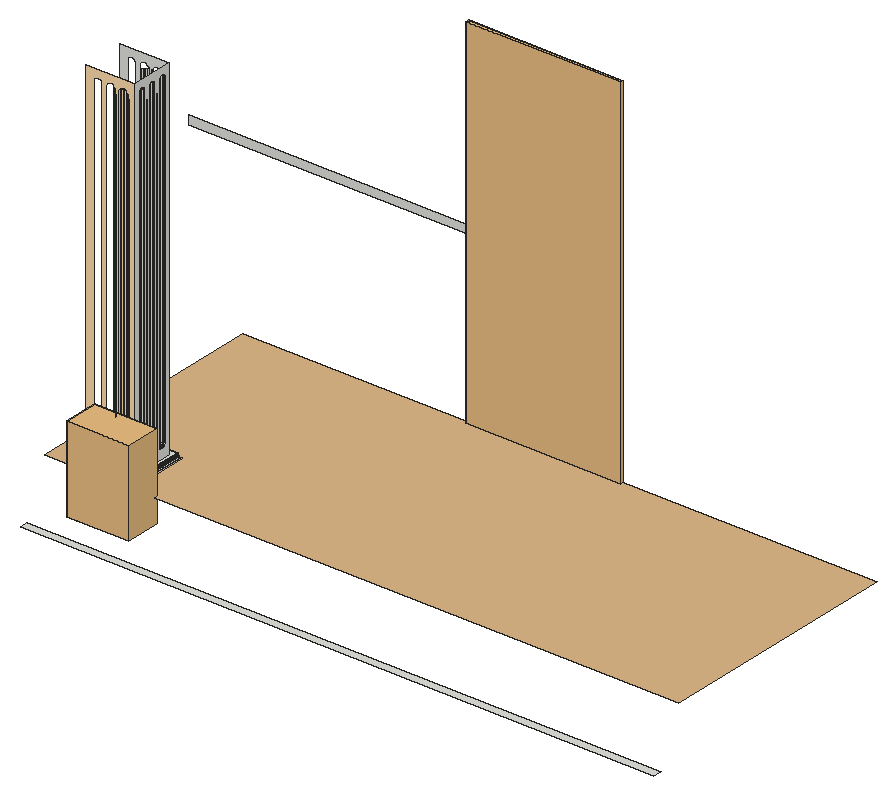
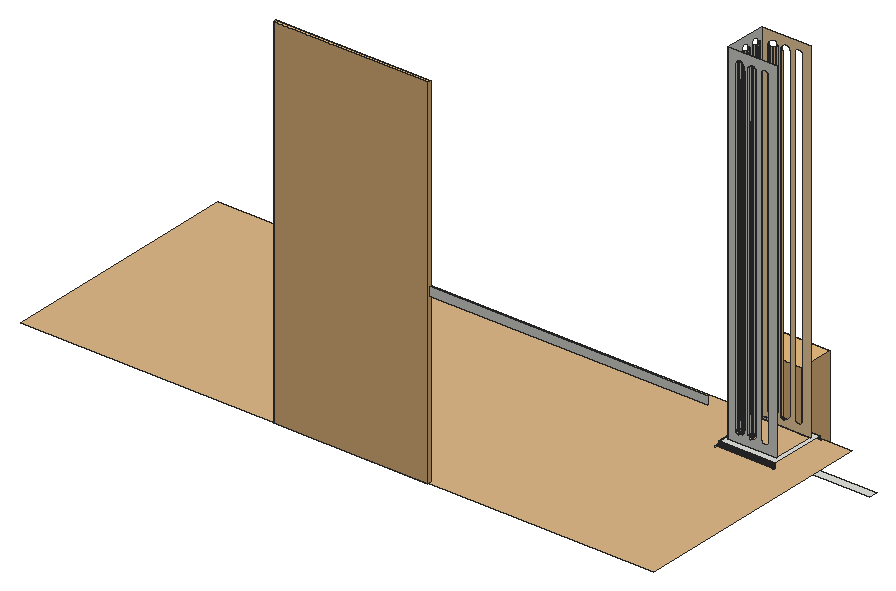
# SketchUp Ruby script. Lengths in inches.
U = 1.inch
M = Sketchup.active_model
def pt(a) = Geom::Point3d.new(a.map { |v| v * U })
def face(e, loops, mat)
  f = e.add_face(loops[0].map { |a| pt(a) })
  loops[1..].each { |l| e.add_face(l.map { |a| pt(a) }).erase! }
  f.material = f.back_material = mat if mat
  f
end
# faces: each face lists its corners as indices into pts; further lists are holes
def faces(e, pts, list, mat = nil) = list.each { |f| face(e, (f[0].is_a?(Array) ? f : [f]).map { |l| l.map { |i| pts[i] } }, mat) }
# xy, xz, yz: faces in a plane at the given z, y or x. An outline is a flat list of corners, or four numbers for a rectangle; further outlines are holes
def ring(l) = l.size == 4 ? [[l[0], l[1]], [l[2], l[1]], [l[2], l[3]], [l[0], l[3]]] : l.each_slice(2).to_a
def flat(e, list, mat, &to3) = list.each { |f| face(e, (f[0].is_a?(Array) ? f : [f]).map { |l| ring(l).map { |u, v| to3.(u, v) } }, mat) }
def xy(e, z, list, mat = nil) = flat(e, list, mat) { |x, y| [x, y, z] }
def xz(e, y, list, mat = nil) = flat(e, list, mat) { |x, z| [x, y, z] }
def yz(e, x, list, mat = nil) = flat(e, list, mat) { |y, z| [x, y, z] }
def lines(e, pts, list) = list.each { |a, b| e.add_line(pt(pts[a]), pt(pts[b])) }
# prism: a flat outline (further loops are holes) pulled along v
def prism(e, loops, v, mat = nil)
  f = face(e, loops, mat); d = Geom::Vector3d.new(v.map { |x| x * U })
  f.pushpull(f.normal.samedirection?(d) ? d.length : -d.length)
end
def box(e, o, s, mat = nil) = prism(e, [[o, [o[0] + s[0], o[1], o[2]], [o[0] + s[0], o[1] + s[1], o[2]], [o[0], o[1] + s[1], o[2]]]], [0, 0, s[2]], mat)
def at(x, y, z, deg = 0) = Geom::Transformation.translation(pt([x, y, z])) * Geom::Transformation.rotation(ORIGIN, Z_AXIS, deg.degrees)
def axes(o, x, y, z) = Geom::Transformation.new([*x, 0, *y, 0, *z, 0, *pt(o).to_a, 1])
def part(name) = M.definitions.add(name)
# library, detail: a bought-in or finely detailed component or shape, given as its bounding box
def library(name, o, s) = part(name).tap { |d| box(d.entities, o, s) }
def detail(e, o, s) = box(e.add_group.entities, o, s)
def put(e, d, t, mat = nil) = e.add_instance(d, t).tap { |i| i.material = mat if mat }
def group(e, t, mat = nil) = e.add_group.tap { |g| g.transformation = t; g.material = mat if mat }.entities
root = M.entities
M.materials.add("[0033_NavajoWhite]").color = [255, 222, 173]
M.materials.add("[0036_BurlyWood]").color = [222, 184, 135]
c1 = library("Flower+pot",[-3.29,-4.11,0],[8.25,8.08,16.09])
c2 = library("Entrance door",[0,0,0],[5.9375,43.31,84.65])
xy(root,0,[[103.43,0,251.04,1.91]])
xy(root,12,[[103.43,7.125,251.04,64.75]],"[0036_BurlyWood]")
xy(root,13.17,[[[110.21,8.1,123.2,21.09],[111,9.67,122.41,19.51]]])
xz(root,8.1,[[110.21,13.02,123.2,13.17]])
xz(root,9.67,[[[111,13.17,122.41,94.95],[113.75,14.97,113.5,15,113.26,15.09,113.06,15.24,112.9,15.42,112.8,15.64,112.77,15.875,112.77,92.25,112.8,92.48,112.9,92.7,113.06,92.89,113.26,93.03,113.5,93.12,113.75,93.15,114.01,93.12,114.25,93.03,114.45,92.89,114.61,92.7,114.7,92.48,114.74,92.25,114.74,15.875,114.7,15.64,114.61,15.42,114.45,15.24,114.25,15.09,114.01,15],[119.66,14.97,119.4,15,119.17,15.09,118.96,15.24,118.81,15.42,118.71,15.64,118.67,15.875,118.67,92.25,118.71,92.48,118.81,92.7,118.96,92.89,119.17,93.03,119.4,93.12,119.66,93.15,119.91,93.12,120.15,93.03,120.35,92.89,120.51,92.7,120.61,92.48,120.64,92.25,120.64,15.875,120.61,15.64,120.51,15.42,120.35,15.24,120.15,15.09,119.91,15],[116.71,14.97,116.45,15,116.21,15.09,116.01,15.24,115.85,15.42,115.76,15.64,115.72,15.875,115.72,92.25,115.76,92.48,115.85,92.7,116.01,92.89,116.21,93.03,116.45,93.12,116.71,93.15,116.96,93.12,117.2,93.03,117.4,92.89,117.56,92.7,117.66,92.48,117.69,92.25,117.69,15.875,117.66,15.64,117.56,15.42,117.4,15.24,117.2,15.09,116.96,15]]],"[0033_NavajoWhite]")
xz(root,19.51,[[[111,13.17,122.41,94.95],[119.66,14.97,119.91,15,120.15,15.09,120.35,15.24,120.51,15.42,120.61,15.64,120.64,15.875,120.64,92.25,120.61,92.48,120.51,92.7,120.35,92.89,120.15,93.03,119.91,93.12,119.66,93.15,119.4,93.12,119.17,93.03,118.96,92.89,118.81,92.7,118.71,92.48,118.67,92.25,118.67,15.875,118.71,15.64,118.81,15.42,118.96,15.24,119.17,15.09,119.4,15],[113.75,14.97,114.01,15,114.25,15.09,114.45,15.24,114.61,15.42,114.7,15.64,114.74,15.875,114.74,92.25,114.7,92.48,114.61,92.7,114.45,92.89,114.25,93.03,114.01,93.12,113.75,93.15,113.5,93.12,113.26,93.03,113.06,92.89,112.9,92.7,112.8,92.48,112.77,92.25,112.77,15.875,112.8,15.64,112.9,15.42,113.06,15.24,113.26,15.09,113.5,15],[116.71,14.97,116.96,15,117.2,15.09,117.4,15.24,117.56,15.42,117.66,15.64,117.69,15.875,117.69,92.25,117.66,92.48,117.56,92.7,117.4,92.89,117.2,93.03,116.96,93.12,116.71,93.15,116.45,93.12,116.21,93.03,116.01,92.89,115.85,92.7,115.76,92.48,115.72,92.25,115.72,15.875,115.76,15.64,115.85,15.42,116.01,15.24,116.21,15.09,116.45,15]]])
xz(root,21.09,[[110.21,13.02,123.2,13.17]])
xz(root,64.75,[[155.99,12,191.99,38.25],[155.99,38.25,191.99,51.19],[90.9,51.19,155.99,53.19],[155.99,51.19,191.99,53.19],[155.99,53.19,191.99,93.75]])
yz(root,122.41,[[[9.67,13.17,19.51,94.95],[17.55,15.23,17.29,15.27,17.05,15.36,16.85,15.5,16.69,15.69,16.59,15.9,16.5625,16.14,16.5625,92.51,16.59,92.74,16.69,92.96,16.85,93.15,17.05,93.29,17.29,93.38,17.55,93.41,17.8,93.38,18.04,93.29,18.24,93.15,18.4,92.96,18.5,92.74,18.53,92.51,18.53,16.14,18.5,15.9,18.4,15.69,18.24,15.5,18.04,15.36,17.8,15.27],[14.59,15.23,14.34,15.27,14.1,15.36,13.9,15.5,13.74,15.69,13.64,15.9,13.61,16.14,13.61,92.51,13.64,92.74,13.74,92.96,13.9,93.15,14.1,93.29,14.34,93.38,14.59,93.41,14.85,93.38,15.08,93.29,15.29,93.15,15.44,92.96,15.54,92.74,15.58,92.51,15.58,16.14,15.54,15.9,15.44,15.69,15.29,15.5,15.08,15.36,14.85,15.27],[11.64,15.23,11.39,15.27,11.15,15.36,10.94,15.5,10.79,15.69,10.6875,15.9,10.66,16.14,10.66,92.51,10.6875,92.74,10.79,92.96,10.94,93.15,11.15,93.29,11.39,93.38,11.64,93.41,11.89,93.38,12.13,93.29,12.34,93.15,12.49,92.96,12.59,92.74,12.625,92.51,12.625,16.14,12.59,15.9,12.49,15.69,12.34,15.5,12.13,15.36,11.89,15.27]]])
yz(root,123.2,[[8.1,12.13,21.09,13.02],[8.1,13.02,21.09,13.17]])
yz(root,123.72,[[7.58,11.46,21.61,12.13]])
p = [[123.55,7.74,12.13],[123.55,21.44,12.13],[123.52,21.41,12.15],[123.52,7.78,12.15],[123.46,7.84,12.2],[109.95,7.84,12.2],
  [109.89,7.78,12.15],[123.46,21.35,12.2],[109.89,21.41,12.15],[109.95,21.35,12.2],[109.86,21.44,12.13],[123.4,7.9,12.27],
  [110.01,7.9,12.27],[123.4,21.29,12.27],[110.01,21.29,12.27],[123.35,7.95,12.36],[110.0625,7.95,12.36],[123.35,21.24,12.36],
  [110.0625,21.24,12.36],[123.3,8,12.47],[110.11,8,12.47],[123.3,21.1875,12.47],[110.11,21.1875,12.47],[123.26,8.03,12.59],
  [110.15,8.03,12.59],[123.26,21.15,12.59],[110.15,21.15,12.59],[123.23,8.06,12.73],[110.18,8.06,12.73],[123.23,21.12,12.73],
  [110.18,21.12,12.73],[123.21,8.09,12.87],[110.2,8.09,12.87],[123.21,21.1,12.87],[110.2,21.1,12.87],[123.2,8.1,13.02],
  [110.21,8.1,13.02],[123.2,21.09,13.02],[110.21,21.09,13.02],[116.71,9.67,14.97],[116.77,9.92,15],[116.71,9.93,15],
  [116.83,9.89,15],[116.89,9.85,15],[116.93,9.8,15],[116.95,9.74,15],[116.96,9.67,15],[117.18,9.8,15.09],
  [117.13,9.92,15.09],[117.2,9.67,15.09],[119.18,9.8,15.09],[119.17,9.67,15.09],[119.4,9.67,15],[119.41,9.74,15],
  [119.4375,9.8,15],[119.23,9.92,15.09],[119.66,9.67,14.97],[119.48,9.85,15],[119.53,9.89,15],[119.59,9.92,15],
  [119.66,9.93,15],[119.72,9.92,15],[119.79,9.89,15],[119.84,9.85,15],[119.88,9.8,15],[119.9,9.74,15],
  [119.91,9.67,15],[120.13,9.8,15.09],[120.08,9.92,15.09],[120.15,9.67,15.09],[117.05,10.02,15.09],[119.3125,10.02,15.09],
  [120.01,10.02,15.09],[116.83,10.15,15.09],[116.71,10.16,15.09],[116.95,10.1,15.09],[119.41,10.1,15.09],[119.53,10.15,15.09],
  [119.66,10.16,15.09],[119.79,10.15,15.09],[119.9,10.1,15.09],[116.71,19.26,15],[116.71,19.02,15.09],[116.83,19.04,15.09],
  [116.77,19.27,15],[116.95,19.09,15.09],[116.83,19.29,15],[119.53,19.29,15],[119.41,19.09,15.09],[119.53,19.04,15.09],
  [119.59,19.27,15],[119.66,19.02,15.09],[119.66,19.26,15],[119.79,19.04,15.09],[119.72,19.27,15],[119.9,19.09,15.09],
  [119.79,19.29,15],[117.05,19.17,15.09],[116.89,19.33,15],[119.48,19.33,15],[119.3125,19.17,15.09],[120.01,19.17,15.09],
  [119.84,19.33,15],[117.13,19.27,15.09],[116.93,19.39,15],[119.4375,19.39,15],[119.23,19.27,15.09],[120.08,19.27,15.09],
  [119.88,19.39,15],[116.71,19.51,14.97],[117.18,19.39,15.09],[116.95,19.45,15],[119.41,19.45,15],[119.18,19.39,15.09],
  [119.66,19.51,14.97],[120.13,19.39,15.09],[119.9,19.45,15],[116.96,19.51,15],[117.2,19.51,15.09],[119.4,19.51,15],
  [119.17,19.51,15.09],[119.91,19.51,15],[120.15,19.51,15.09],[117.4,9.67,15.24],[117.38,9.85,15.24],[118.99,9.85,15.24],
  [118.96,9.67,15.24],[120.35,9.67,15.24],[120.33,9.85,15.24],[117.31,10.02,15.24],[119.06,10.02,15.24],[120.26,10.02,15.24],
  [117.2,10.16,15.24],[119.17,10.16,15.24],[120.15,10.16,15.24],[117.05,10.27,15.24],[119.3125,10.27,15.24],[120.01,10.27,15.24],
  [116.89,10.34,15.24],[116.71,10.37,15.24],[119.48,10.34,15.24],[119.66,10.37,15.24],[119.84,10.34,15.24],[116.71,18.82,15.24],
  [116.89,18.84,15.24],[117.05,18.91,15.24],[119.3125,18.91,15.24],[119.48,18.84,15.24],[119.66,18.82,15.24],[119.84,18.84,15.24],
  [120.01,18.91,15.24],[117.2,19.02,15.24],[119.17,19.02,15.24],[120.15,19.02,15.24],[117.31,19.17,15.24],[119.06,19.17,15.24],
  [120.26,19.17,15.24],[117.38,19.33,15.24],[118.99,19.33,15.24],[120.33,19.33,15.24],[117.4,19.51,15.24],[118.96,19.51,15.24],
  [120.35,19.51,15.24],[117.56,9.67,15.42],[117.53,9.89,15.42],[118.84,9.89,15.42],[118.81,9.67,15.42],[120.51,9.67,15.42],
  [120.48,9.89,15.42],[117.44,10.1,15.42],[118.92,10.1,15.42],[120.4,10.1,15.42],[117.31,10.27,15.42],[119.06,10.27,15.42],
  [120.26,10.27,15.42],[117.13,10.41,15.42],[119.23,10.41,15.42],[120.08,10.41,15.42],[116.93,10.49,15.42],[116.71,10.52,15.42],
  [119.4375,10.49,15.42],[119.66,10.52,15.42],[119.88,10.49,15.42],[122.29,11.42,15.27],[122.41,11.64,15.23],[122.23,11.46,15.27],
  [122.35,11.39,15.27],[122.41,11.39,15.27],[122.19,11.51,15.27],[122.17,11.57,15.27],[122.16,11.64,15.27],[122.17,11.71,15.27],
  [122.19,11.77,15.27],[122.23,11.82,15.27],[122.29,11.86,15.27],[122.35,11.89,15.27],[122.41,11.89,15.27],[122.35,14.35,15.27],
  [122.41,14.59,15.23],[122.29,14.37,15.27],[122.41,14.34,15.27],[122.23,14.41,15.27],[122.19,14.47,15.27],[122.17,14.53,15.27],
  [122.16,14.59,15.27],[122.17,14.66,15.27],[122.19,14.72,15.27],[122.23,14.77,15.27],[122.29,14.8125,15.27],[122.35,14.84,15.27],
  [122.41,14.85,15.27],[122.41,17.55,15.23],[122.23,17.37,15.27],[122.29,17.32,15.27],[122.35,17.3,15.27],[122.41,17.29,15.27],
  [122.17,17.48,15.27],[122.19,17.42,15.27],[122.16,17.55,15.27],[122.17,17.61,15.27],[122.19,17.67,15.27],[122.23,17.73,15.27],
  [122.29,17.77,15.27],[122.35,17.79,15.27],[122.41,17.8,15.27],[116.71,18.66,15.42],[116.93,18.69,15.42],[117.13,18.78,15.42],
  [119.23,18.78,15.42],[119.4375,18.69,15.42],[119.66,18.66,15.42],[119.88,18.69,15.42],[120.08,18.78,15.42],[117.31,18.91,15.42],
  [119.06,18.91,15.42],[120.26,18.91,15.42],[117.44,19.09,15.42],[118.92,19.09,15.42],[120.4,19.09,15.42],[117.53,19.29,15.42],
  [118.84,19.29,15.42],[120.48,19.29,15.42],[117.56,19.51,15.42],[118.81,19.51,15.42],[120.51,19.51,15.42],[122.29,11.16,15.36],
  [122.41,11.15,15.36],[122.17,11.21,15.36],[122.07,11.29,15.36],[121.99,11.39,15.36],[121.9375,11.51,15.36],[121.92,11.64,15.36],
  [121.9375,11.77,15.36],[121.99,11.89,15.36],[122.07,11.99,15.36],[122.17,12.07,15.36],[122.29,12.12,15.36],[122.41,12.13,15.36],
  [122.29,14.12,15.36],[122.17,14.17,15.36],[122.41,14.1,15.36],[122.07,14.24,15.36],[121.99,14.35,15.36],[121.9375,14.47,15.36],
  [121.92,14.59,15.36],[121.9375,14.72,15.36],[121.99,14.84,15.36],[122.07,14.94,15.36],[122.17,15.02,15.36],[122.29,15.07,15.36],
  [122.41,15.08,15.36],[122.07,17.2,15.36],[122.17,17.12,15.36],[122.29,17.07,15.36],[122.41,17.05,15.36],[121.99,17.3,15.36],
  [121.9375,17.42,15.36],[121.92,17.55,15.36],[121.9375,17.67,15.36],[121.99,17.79,15.36],[122.07,17.89,15.36],[122.17,17.97,15.36],
  [122.29,18.02,15.36],[122.41,18.04,15.36],[117.66,9.67,15.64],[117.625,9.92,15.64],[118.74,9.92,15.64],[118.71,9.67,15.64],
  [120.61,9.67,15.64],[120.58,9.92,15.64],[117.53,10.15,15.64],[118.84,10.15,15.64],[120.48,10.15,15.64],[117.38,10.34,15.64],
  [118.99,10.34,15.64],[120.33,10.34,15.64],[117.18,10.49,15.64],[119.18,10.49,15.64],[120.13,10.49,15.64],[116.95,10.59,15.64],
  [119.41,10.59,15.64],[119.9,10.59,15.64],[116.71,10.62,15.64],[119.66,10.62,15.64],[122.23,10.97,15.5],[122.41,10.94,15.5],
  [122.07,11.04,15.5],[121.92,11.15,15.5],[121.8125,11.29,15.5],[121.74,11.46,15.5],[121.72,11.64,15.5],[121.74,11.82,15.5],
  [121.8125,11.99,15.5],[121.92,12.13,15.5],[122.07,12.24,15.5],[122.23,12.3125,15.5],[122.41,12.34,15.5],[122.23,13.92,15.5],
  [122.07,13.99,15.5],[122.41,13.9,15.5],[121.92,14.1,15.5],[121.8125,14.24,15.5],[121.74,14.41,15.5],[121.72,14.59,15.5],
  [121.74,14.77,15.5],[121.8125,14.94,15.5],[121.92,15.08,15.5],[122.07,15.2,15.5],[122.23,15.26,15.5],[122.41,15.29,15.5],
  [122.23,16.875,15.5],[122.41,16.85,15.5],[121.92,17.05,15.5],[122.07,16.94,15.5],[121.8125,17.2,15.5],[121.74,17.37,15.5],
  [121.72,17.55,15.5],[121.74,17.73,15.5],[121.8125,17.89,15.5],[121.92,18.04,15.5],[122.07,18.15,15.5],[122.23,18.22,15.5],
  [122.41,18.24,15.5],[116.71,18.5625,15.64],[116.95,18.6,15.64],[117.18,18.69,15.64],[119.18,18.69,15.64],[119.41,18.6,15.64],
  [119.66,18.5625,15.64],[119.9,18.6,15.64],[120.13,18.69,15.64],[117.38,18.84,15.64],[118.99,18.84,15.64],[120.33,18.84,15.64],
  [117.53,19.04,15.64],[118.84,19.04,15.64],[120.48,19.04,15.64],[117.625,19.27,15.64],[118.74,19.27,15.64],[120.58,19.27,15.64],
  [117.66,19.51,15.64],[118.71,19.51,15.64],[120.61,19.51,15.64],[122.19,10.82,15.69],[121.99,10.9,15.69],[122.41,10.79,15.69],
  [121.8125,11.04,15.69],[121.68,11.21,15.69],[121.59,11.42,15.69],[121.5625,11.64,15.69],[121.59,11.86,15.69],[121.68,12.07,15.69],
  [121.8125,12.24,15.69],[121.99,12.38,15.69],[122.19,12.46,15.69],[122.41,12.49,15.69],[122.19,13.77,15.69],[122.41,13.74,15.69],
  [121.99,13.85,15.69],[121.8125,13.99,15.69],[121.68,14.17,15.69],[121.59,14.37,15.69],[121.5625,14.59,15.69],[121.59,14.8125,15.69],
  [121.68,15.02,15.69],[121.8125,15.2,15.69],[121.99,15.33,15.69],[122.19,15.42,15.69],[122.41,15.44,15.69],[121.99,16.81,15.69],
  [122.19,16.72,15.69],[122.41,16.69,15.69],[121.8125,16.94,15.69],[121.68,17.12,15.69],[121.59,17.32,15.69],[121.5625,17.55,15.69],
  [121.59,17.77,15.69],[121.68,17.97,15.69],[121.8125,18.15,15.69],[121.99,18.28,15.69],[122.19,18.37,15.69],[122.41,18.4,15.69],
  [117.69,9.67,15.875],[117.66,9.93,15.875],[118.71,9.93,15.875],[118.67,9.67,15.875],[120.64,9.67,15.875],[120.61,9.93,15.875],
  [117.56,10.16,15.875],[118.81,10.16,15.875],[120.51,10.16,15.875],[117.4,10.37,15.875],[118.96,10.37,15.875],[120.35,10.37,15.875],
  [117.2,10.52,15.875],[119.17,10.52,15.875],[120.15,10.52,15.875],[116.96,10.62,15.875],[119.4,10.62,15.875],[119.91,10.62,15.875],
  [116.71,10.66,15.875],[119.66,10.66,15.875],[116.71,18.53,15.875],[116.96,18.5625,15.875],[119.4,18.5625,15.875],[119.66,18.53,15.875],
  [119.91,18.5625,15.875],[117.2,18.66,15.875],[119.17,18.66,15.875],[120.15,18.66,15.875],[117.4,18.82,15.875],[118.96,18.82,15.875],
  [120.35,18.82,15.875],[117.56,19.02,15.875],[118.81,19.02,15.875],[120.51,19.02,15.875],[117.66,19.26,15.875],[118.71,19.26,15.875],
  [120.61,19.26,15.875],[117.69,19.51,15.875],[118.67,19.51,15.875],[120.64,19.51,15.875],[122.17,10.72,15.9],[121.9375,10.82,15.9],
  [122.41,10.6875,15.9],[121.74,10.97,15.9],[121.59,11.16,15.9],[121.5,11.39,15.9],[121.46,11.64,15.9],[121.5,11.89,15.9],
  [121.59,12.12,15.9],[121.74,12.3125,15.9],[121.9375,12.46,15.9],[122.17,12.56,15.9],[122.41,12.59,15.9],[122.17,13.67,15.9],
  [122.41,13.64,15.9],[121.9375,13.77,15.9],[121.74,13.92,15.9],[121.59,14.12,15.9],[121.5,14.35,15.9],[121.46,14.59,15.9],
  [121.5,14.84,15.9],[121.59,15.07,15.9],[121.74,15.26,15.9],[121.9375,15.42,15.9],[122.17,15.51,15.9],[122.41,15.54,15.9],
  [121.9375,16.72,15.9],[122.17,16.625,15.9],[122.41,16.59,15.9],[121.74,16.875,15.9],[121.59,17.07,15.9],[121.5,17.3,15.9],
  [121.46,17.55,15.9],[121.5,17.79,15.9],[121.59,18.02,15.9],[121.74,18.22,15.9],[121.9375,18.37,15.9],[122.17,18.46,15.9],
  [122.41,18.5,15.9],[117.69,9.67,92.25],[117.66,9.93,92.25],[118.71,9.93,92.25],[118.67,9.67,92.25],[120.64,9.67,92.25],
  [120.61,9.93,92.25],[117.56,10.16,92.25],[118.81,10.16,92.25],[120.51,10.16,92.25],[117.4,10.37,92.25],[118.96,10.37,92.25],
  [120.35,10.37,92.25],[117.2,10.52,92.25],[119.17,10.52,92.25],[120.15,10.52,92.25],[116.96,10.62,92.25],[119.4,10.62,92.25],
  [119.91,10.62,92.25],[116.71,10.66,92.25],[119.66,10.66,92.25],[122.16,10.6875,16.14],[121.92,10.79,16.14],[122.41,10.66,16.14],
  [121.72,10.94,16.14],[121.5625,11.15,16.14],[121.46,11.39,16.14],[121.43,11.64,16.14],[121.46,11.89,16.14],[121.5625,12.13,16.14],
  [121.72,12.34,16.14],[121.92,12.49,16.14],[122.16,12.59,16.14],[122.41,12.625,16.14],[122.16,13.64,16.14],[121.92,13.74,16.14],
  [122.41,13.61,16.14],[121.72,13.9,16.14],[121.5625,14.1,16.14],[121.46,14.34,16.14],[121.43,14.59,16.14],[121.46,14.85,16.14],
  [121.5625,15.08,16.14],[121.72,15.29,16.14],[121.92,15.44,16.14],[122.16,15.54,16.14],[122.41,15.58,16.14],[121.92,16.69,16.14],
  [122.16,16.59,16.14],[122.41,16.5625,16.14],[121.72,16.85,16.14],[121.5625,17.05,16.14],[121.46,17.29,16.14],[121.43,17.55,16.14],
  [121.46,17.8,16.14],[121.5625,18.04,16.14],[121.72,18.24,16.14],[121.92,18.4,16.14],[122.16,18.5,16.14],[116.71,18.53,92.25],
  [116.96,18.5625,92.25],[119.4,18.5625,92.25],[119.66,18.53,92.25],[119.91,18.5625,92.25],[122.41,18.53,16.14],[117.2,18.66,92.25],
  [119.17,18.66,92.25],[120.15,18.66,92.25],[117.4,18.82,92.25],[118.96,18.82,92.25],[120.35,18.82,92.25],[117.56,19.02,92.25],
  [118.81,19.02,92.25],[120.51,19.02,92.25],[117.66,19.26,92.25],[118.71,19.26,92.25],[120.61,19.26,92.25],[117.69,19.51,92.25],
  [118.67,19.51,92.25],[120.64,19.51,92.25],[121.92,10.79,92.51],[122.16,10.6875,92.51],[122.41,10.66,92.51],[121.72,10.94,92.51],
  [121.5625,11.15,92.51],[121.46,11.39,92.51],[121.43,11.64,92.51],[121.46,11.89,92.51],[121.5625,12.13,92.51],[121.72,12.34,92.51],
  [121.92,12.49,92.51],[122.16,12.59,92.51],[122.41,12.625,92.51],[121.92,13.74,92.51],[122.16,13.64,92.51],[122.41,13.61,92.51],
  [121.72,13.9,92.51],[121.5625,14.1,92.51],[121.46,14.34,92.51],[121.43,14.59,92.51],[121.46,14.85,92.51],[121.5625,15.08,92.51],
  [121.72,15.29,92.51],[121.92,15.44,92.51],[122.16,15.54,92.51],[122.41,15.58,92.51],[121.92,16.69,92.51],[122.16,16.59,92.51],
  [122.41,16.5625,92.51],[121.72,16.85,92.51],[121.5625,17.05,92.51],[121.46,17.29,92.51],[121.43,17.55,92.51],[121.46,17.8,92.51],
  [121.5625,18.04,92.51],[121.72,18.24,92.51],[121.92,18.4,92.51],[122.16,18.5,92.51],[122.41,18.53,92.51]]
faces(root,p,[[0,1,2,3],[3,4,5,6],[3,2,7,4],[8,9,7,2],[10,8,2,1],[4,11,12,5],[4,7,13,11],[9,14,13,7],
  [11,15,16,12],[11,13,17,15],[14,18,17,13],[15,19,20,16],[15,17,21,19],[18,22,21,17],[19,23,24,20],[19,21,25,23],
  [22,26,25,21],[23,27,28,24],[23,25,29,27],[26,30,29,25],[27,31,32,28],[27,29,33,31],[30,34,33,29],[31,35,36,32],
  [31,33,37,35],[34,38,37,33],[81,82,83,84],[84,83,85,86],[87,88,89,90],[90,89,91,92],[92,91,93,94],[94,93,95,96],
  [86,85,97,98],[99,100,88,87],[96,95,101,102],[98,97,103,104],[105,106,100,99],[102,101,107,108],[109,81,84],[109,84,86],
  [109,86,98],[109,98,104],[104,103,110,111],[112,113,106,105],[114,105,99],[114,99,87],[114,87,90],[114,90,92],
  [114,92,94],[114,94,96],[114,96,102],[114,102,108],[108,107,115,116],[109,104,111],[111,117,109],[110,118,117,111],
  [112,119,120,113],[112,114,119],[114,112,105],[114,108,116],[116,121,114],[115,122,121,116],[82,143,144,83],[83,144,145,85],
  [88,146,147,89],[89,147,148,91],[91,148,149,93],[93,149,150,95],[85,145,151,97],[100,152,146,88],[95,150,153,101],[97,151,154,103],
  [106,155,152,100],[101,153,156,107],[103,154,157,110],[113,158,155,106],[107,156,159,115],[157,160,118,110],[113,120,161,158],[159,162,122,115],
  [183,184,185],[186,184,183],[184,186,187],[188,184,189],[185,184,188],[190,184,191],[189,184,190],[191,184,192],
  [192,184,193],[193,184,194],[194,184,195],[196,195,184],[197,198,199],[198,197,200],[201,198,202],[199,198,201],
  [203,198,204],[202,198,203],[204,198,205],[205,198,206],[206,198,207],[207,198,208],[208,198,209],[210,209,198],
  [211,212,213],[211,213,214],[214,215,211],[211,216,217],[211,217,212],[211,218,216],[211,219,218],[211,220,219],
  [211,221,220],[211,222,221],[211,223,222],[223,211,224],[143,225,226,144],[144,226,227,145],[146,228,229,147],[147,229,230,148],
  [148,230,231,149],[149,231,232,150],[145,227,233,151],[152,234,228,146],[150,232,235,153],[151,233,236,154],[155,237,234,152],[153,235,238,156],
  [154,236,239,157],[158,240,237,155],[156,238,241,159],[239,242,160,157],[158,161,243,240],[241,244,162,159],[187,186,245,246],[247,183,185,248],
  [245,186,183,247],[248,185,188,249],[249,188,189,250],[250,189,190,251],[251,190,191,252],[252,191,192,253],[253,192,193,254],[254,193,194,255],
  [255,194,195,256],[257,256,195,196],[258,197,199,259],[200,197,258,260],[261,201,202,262],[259,199,201,261],[262,202,203,263],[263,203,204,264],
  [264,204,205,265],[265,205,206,266],[266,206,207,267],[267,207,208,268],[268,208,209,269],[270,269,209,210],[212,271,272,213],[213,272,273,214],
  [273,274,215,214],[217,275,271,212],[216,276,275,217],[218,277,276,216],[219,278,277,218],[220,279,278,219],[221,280,279,220],[222,281,280,221],
  [223,282,281,222],[223,224,283,282],[246,245,304,305],[306,247,248,307],[304,245,247,306],[307,248,249,308],[308,249,250,309],[309,250,251,310],
  [310,251,252,311],[311,252,253,312],[312,253,254,313],[313,254,255,314],[314,255,256,315],[316,315,256,257],[317,258,259,318],[260,258,317,319],
  [318,259,261,320],[320,261,262,321],[321,262,263,322],[322,263,264,323],[323,264,265,324],[324,265,266,325],[325,266,267,326],[326,267,268,327],
  [327,268,269,328],[329,328,269,270],[330,331,274,273],[271,332,333,272],[272,333,330,273],[275,334,332,271],[276,335,334,275],[277,336,335,276],
  [278,337,336,277],[279,338,337,278],[280,339,338,279],[281,340,339,280],[282,341,340,281],[282,283,342,341],[225,343,344,226],[226,344,345,227],
  [228,346,347,229],[229,347,348,230],[230,348,349,231],[231,349,350,232],[227,345,351,233],[234,352,346,228],[232,350,353,235],[233,351,354,236],
  [237,355,352,234],[235,353,356,238],[236,354,357,239],[240,358,355,237],[238,356,359,241],[357,360,242,239],[240,243,361,358],[359,362,244,241],
  [363,304,306,364],[305,304,363,365],[364,306,307,366],[366,307,308,367],[367,308,309,368],[368,309,310,369],[369,310,311,370],[370,311,312,371],
  [371,312,313,372],[372,313,314,373],[373,314,315,374],[375,374,315,316],[319,317,376,377],[376,317,318,378],[378,318,320,379],[379,320,321,380],
  [380,321,322,381],[381,322,323,382],[382,323,324,383],[383,324,325,384],[384,325,326,385],[385,326,327,386],[386,327,328,387],[388,387,328,329],
  [333,389,390,330],[390,391,331,330],[332,392,389,333],[334,393,392,332],[335,394,393,334],[336,395,394,335],[337,396,395,336],[338,397,396,337],
  [339,398,397,338],[340,399,398,339],[341,400,399,340],[341,342,401,400],[343,422,423,344],[347,424,425,348],[348,425,426,349],[344,423,427,345],
  [346,428,424,347],[349,426,429,350],[345,427,430,351],[352,431,428,346],[350,429,432,353],[351,430,433,354],[355,434,431,352],[353,432,435,356],
  [354,433,436,357],[358,437,434,355],[356,435,438,359],[436,439,360,357],[358,361,440,437],[438,441,362,359],[442,363,364,443],[365,363,442,444],
  [443,364,366,445],[445,366,367,446],[446,367,368,447],[447,368,369,448],[448,369,370,449],[449,370,371,450],[450,371,372,451],[451,372,373,452],
  [452,373,374,453],[454,453,374,375],[377,376,455,456],[455,376,378,457],[457,378,379,458],[458,379,380,459],[459,380,381,460],[460,381,382,461],
  [461,382,383,462],[462,383,384,463],[463,384,385,464],[464,385,386,465],[465,386,387,466],[467,466,387,388],[389,468,469,390],[469,470,391,390],
  [392,471,468,389],[393,472,471,392],[394,473,472,393],[395,474,473,394],[396,475,474,395],[397,476,475,396],[398,477,476,397],[399,478,477,398],
  [400,479,478,399],[400,401,480,479],[501,442,443,502],[444,442,501,503],[502,443,445,504],[504,445,446,505],[505,446,447,506],[506,447,448,507],
  [507,448,449,508],[508,449,450,509],[509,450,451,510],[510,451,452,511],[511,452,453,512],[513,512,453,454],[514,455,457,515],[456,455,514,516],
  [515,457,458,517],[517,458,459,518],[518,459,460,519],[519,460,461,520],[520,461,462,521],[521,462,463,522],[522,463,464,523],[523,464,465,524],
  [524,465,466,525],[526,525,466,467],[468,527,528,469],[528,529,470,469],[471,530,527,468],[472,531,530,471],[473,532,531,472],[474,533,532,473],
  [475,534,533,474],[476,535,534,475],[477,536,535,476],[478,537,536,477],[479,538,537,478],[423,422,539,540],[425,424,541,542],[426,425,542,543],
  [479,480,544,538],[427,423,540,545],[424,428,546,541],[429,426,543,547],[430,427,545,548],[428,431,549,546],[432,429,547,550],[433,430,548,551],
  [431,434,552,549],[435,432,550,553],[436,433,551,554],[434,437,555,552],[438,435,553,556],[439,436,554,557],[437,440,558,555],[441,438,556,559],
  [501,502,560,561],[503,501,561,562],[502,504,563,560],[504,505,564,563],[505,506,565,564],[506,507,566,565],[507,508,567,566],[508,509,568,567],
  [509,510,569,568],[510,511,570,569],[511,512,571,570],[512,513,572,571],[514,515,573,574],[516,514,574,575],[515,517,576,573],[517,518,577,576],
  [518,519,578,577],[519,520,579,578],[520,521,580,579],[521,522,581,580],[522,523,582,581],[523,524,583,582],[524,525,584,583],[525,526,585,584],
  [528,527,586,587],[529,528,587,588],[527,530,589,586],[530,531,590,589],[531,532,591,590],[532,533,592,591],[533,534,593,592],[534,535,594,593],
  [535,536,595,594],[536,537,596,595],[537,538,597,596],[538,544,598,597]])
faces(root,p,[[39,40,41],[39,42,40],[39,43,42],[39,44,43],[39,45,44],[45,39,46],[45,47,48,44],[45,46,49,47],
  [50,51,52,53],[54,55,50,53],[53,52,56],[56,54,53],[56,57,54],[56,58,57],[56,59,58],[56,60,59],
  [56,61,60],[56,62,61],[56,63,62],[56,64,63],[56,65,64],[65,56,66],[65,67,68,64],[65,66,69,67],
  [44,48,70,43],[57,71,55,54],[64,68,72,63],[40,73,74,41],[42,75,73,40],[43,70,75,42],[58,76,71,57],[59,77,76,58],
  [60,78,77,59],[61,79,78,60],[62,80,79,61],[63,72,80,62],[47,49,123,124],[125,126,51,50],[67,69,127,128],[47,124,129,48],
  [55,130,125,50],[67,128,131,68],[48,129,132,70],[71,133,130,55],[68,131,134,72],[70,132,135,75],[76,136,133,71],[72,134,137,80],
  [73,138,139,74],[75,135,138,73],[77,140,136,76],[78,141,140,77],[79,142,141,78],[80,137,142,79],[124,123,163,164],[165,166,126,125],
  [128,127,167,168],[124,164,169,129],[130,170,165,125],[128,168,171,131],[129,169,172,132],[133,173,170,130],[131,171,174,134],[132,172,175,135],
  [136,176,173,133],[134,174,177,137],[138,178,179,139],[135,175,178,138],[140,180,176,136],[141,181,180,140],[142,182,181,141],[137,177,182,142],
  [164,163,284,285],[286,287,166,165],[168,167,288,289],[164,285,290,169],[170,291,286,165],[168,289,292,171],[169,290,293,172],[173,294,291,170],
  [171,292,295,174],[172,293,296,175],[176,297,294,173],[174,295,298,177],[175,296,299,178],[180,300,297,176],[177,298,301,182],[178,299,302,179],
  [181,303,300,180],[182,301,303,181],[285,284,402,403],[404,405,287,286],[289,288,406,407],[285,403,408,290],[291,409,404,286],[289,407,410,292],
  [290,408,411,293],[294,412,409,291],[292,410,413,295],[293,411,414,296],[297,415,412,294],[295,413,416,298],[296,414,417,299],[300,418,415,297],
  [298,416,419,301],[299,417,420,302],[303,421,418,300],[301,419,421,303],[403,402,481,482],[405,404,483,484],[407,406,485,486],[408,403,482,487],
  [404,409,488,483],[410,407,486,489],[411,408,487,490],[409,412,491,488],[413,410,489,492],[414,411,490,493],[412,415,494,491],[416,413,492,495],
  [417,414,493,496],[415,418,497,494],[419,416,495,498],[420,417,496,499],[418,421,500,497],[421,419,498,500]],"[0033_NavajoWhite]")
put(root,c1,axes([120.06,4.11,6],[1.76453,0,0],[0,1,0],[0,0,1.24]))
put(root,c2,axes([155.99,64.87,12],[0,-0.12143,0],[0.8296,0,0],[0,0,0.98979]))
